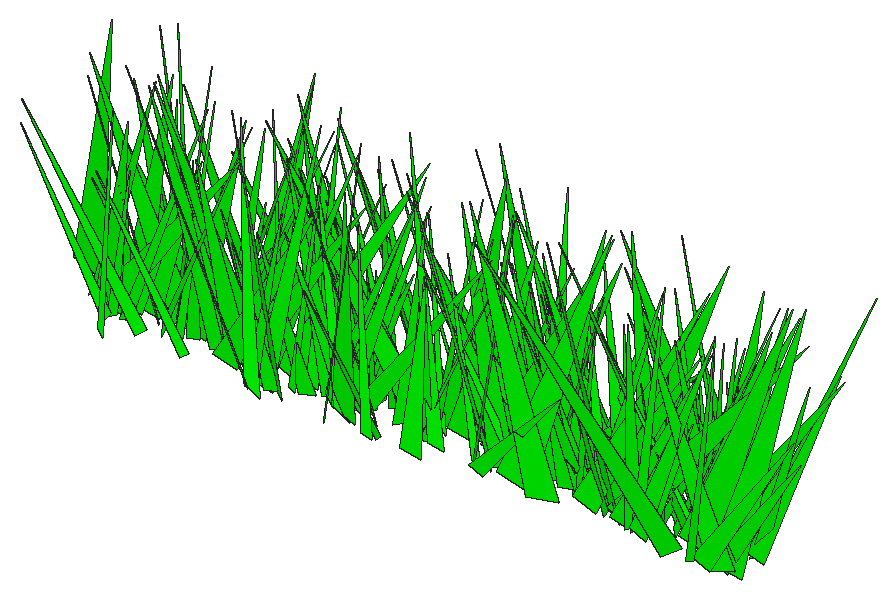
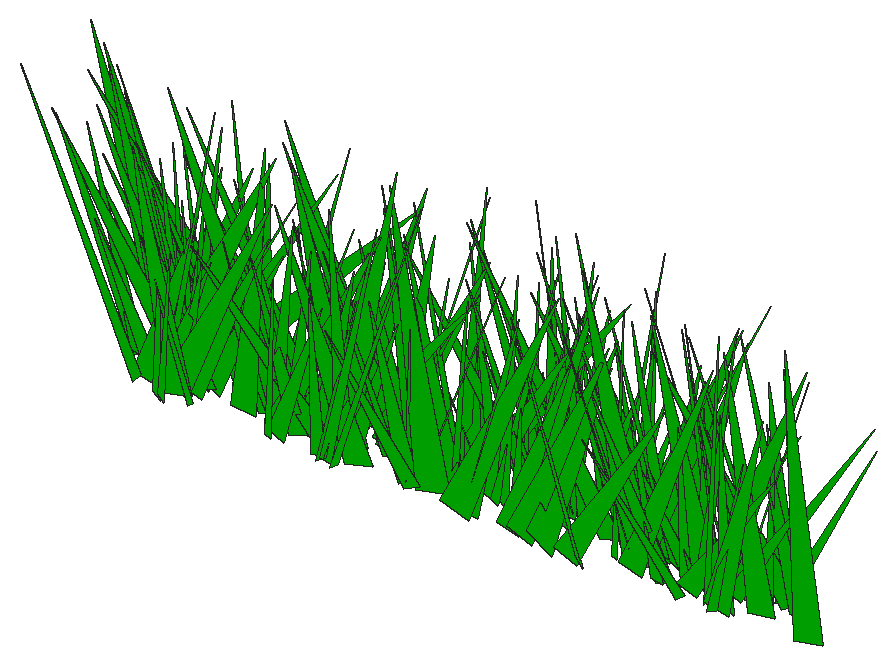
# SketchUp Ruby script. Lengths in inches.
U = 1.inch
M = Sketchup.active_model
def pt(a) = Geom::Point3d.new(a.map { |v| v * U })
def face(e, loops, mat)
  f = e.add_face(loops[0].map { |a| pt(a) })
  loops[1..].each { |l| e.add_face(l.map { |a| pt(a) }).erase! }
  f.material = f.back_material = mat if mat
  f
end
# faces: each face lists its corners as indices into pts; further lists are holes
def faces(e, pts, list, mat = nil) = list.each { |f| face(e, (f[0].is_a?(Array) ? f : [f]).map { |l| l.map { |i| pts[i] } }, mat) }
# xy, xz, yz: faces in a plane at the given z, y or x. An outline is a flat list of corners, or four numbers for a rectangle; further outlines are holes
def ring(l) = l.size == 4 ? [[l[0], l[1]], [l[2], l[1]], [l[2], l[3]], [l[0], l[3]]] : l.each_slice(2).to_a
def flat(e, list, mat, &to3) = list.each { |f| face(e, (f[0].is_a?(Array) ? f : [f]).map { |l| ring(l).map { |u, v| to3.(u, v) } }, mat) }
def xy(e, z, list, mat = nil) = flat(e, list, mat) { |x, y| [x, y, z] }
def xz(e, y, list, mat = nil) = flat(e, list, mat) { |x, z| [x, y, z] }
def yz(e, x, list, mat = nil) = flat(e, list, mat) { |y, z| [x, y, z] }
def lines(e, pts, list) = list.each { |a, b| e.add_line(pt(pts[a]), pt(pts[b])) }
# prism: a flat outline (further loops are holes) pulled along v
def prism(e, loops, v, mat = nil)
  f = face(e, loops, mat); d = Geom::Vector3d.new(v.map { |x| x * U })
  f.pushpull(f.normal.samedirection?(d) ? d.length : -d.length)
end
def box(e, o, s, mat = nil) = prism(e, [[o, [o[0] + s[0], o[1], o[2]], [o[0] + s[0], o[1] + s[1], o[2]], [o[0], o[1] + s[1], o[2]]]], [0, 0, s[2]], mat)
def at(x, y, z, deg = 0) = Geom::Transformation.translation(pt([x, y, z])) * Geom::Transformation.rotation(ORIGIN, Z_AXIS, deg.degrees)
def axes(o, x, y, z) = Geom::Transformation.new([*x, 0, *y, 0, *z, 0, *pt(o).to_a, 1])
def part(name) = M.definitions.add(name)
# library, detail: a bought-in or finely detailed component or shape, given as its bounding box
def library(name, o, s) = part(name).tap { |d| box(d.entities, o, s) }
def detail(e, o, s) = box(e.add_group.entities, o, s)
def put(e, d, t, mat = nil) = e.add_instance(d, t).tap { |i| i.material = mat if mat }
def group(e, t, mat = nil) = e.add_group.tap { |g| g.transformation = t; g.material = mat if mat }.entities
root = M.entities
M.materials.add("[0065_Lime]").color = [0, 255, 0]
c1 = part("fur_instance\#9")
p = [[0.8125,0,1.79],[0.67,-0.02,1.48],[0,-0.11,0],[0,0.11,0]]
faces(c1.entities,p,[[0,1,2,3]])
put(root,c1,axes([147.4375,26.02,1.48],[-5.64516,0.3336,1.45571],[-2.08323,-0.82888,1.01979],[2.12109,0.07376,4.87587]),"[0065_Lime]")
put(root,c1,axes([145.2,25.94,1.48],[8.40795,0.23314,2.16306],[-1.12337,1.22283,-1.52742],[-2.92617,0.20046,6.80163]),"[0065_Lime]")
put(root,c1,axes([165.61,26.26,1.48],[2.66875,-0.65598,0.87046],[4.49426,0.28351,-1.95751],[1.65526,0.28786,3.91148]),"[0065_Lime]")
put(root,c1,axes([142.26,26.54,1.48],[-8.02336,-0.38155,1.65588],[2.34325,-1.15401,-1.39815],[2.45487,-0.14551,6.74656]),"[0065_Lime]")
put(root,c1,axes([147.97,26.21,1.48],[-3.82032,-0.24279,0.04351],[1.61672,-0.49536,1.29689],[-0.61201,0.20701,3.15435]),"[0065_Lime]")
put(root,c1,axes([140.84,26.17,1.48],[-9.03308,-0.11216,0.2971],[0.85058,-1.24949,1.30518],[0.21674,0.22922,7.25986]),"[0065_Lime]")
put(root,c1,axes([164,26.24,1.48],[-6.04067,-0.94159,0.54512],[5.82851,-0.66764,4.0909],[-3.37327,0.53256,6.0923]),"[0065_Lime]")
put(root,c1,axes([132.93,25.9375,1.48],[6.59499,0.11964,2.32533],[0.40682,0.92959,-2.36602],[-2.95495,0.39499,4.86404]),"[0065_Lime]")
put(root,c1,axes([149.88,26.03,1.48],[-2.46962,0.72649,0.09041],[-5.01732,-0.34081,1.08686],[1.2525,0.06724,4.53207]),"[0065_Lime]")
put(root,c1,axes([166.41,26.53,1.48],[1.55477,-0.64987,0.45687],[4.2566,0.16434,-1.75131],[1.89367,0.16417,3.5615]),"[0065_Lime]")
put(root,c1,axes([145.53,26.86,1.48],[-4.02699,-0.94749,0.69367],[6.4082,-0.57572,-1.73659],[2.26451,-0.05572,6.14783]),"[0065_Lime]")
put(root,c1,axes([165.06,26.21,1.48],[5.85886,0.44745,1.24971],[-2.77667,0.84099,-1.47688],[-2.18863,0.13084,5.21912]),"[0065_Lime]")
put(root,c1,axes([166.75,26.49,1.48],[4.8644,-1.02334,2.31887],[7.81718,0.62202,-1.65156],[0.23532,0.49069,6.92962]),"[0065_Lime]")
put(root,c1,axes([153,26.61,1.48],[1.4391,-0.53575,0.3117],[3.28378,0.14278,-1.80769],[1.97492,0.15299,2.77859]),"[0065_Lime]")
put(root,c1,axes([166.7,26.33,1.48],[-0.36588,0.97693,0.95814],[-6.61726,0.00969,-2.00296],[-2.43605,-0.17305,5.2969]),"[0065_Lime]")
put(root,c1,axes([141.83,26.59,1.48],[-0.87819,0.53517,1.2943],[-4.04294,-0.06547,-0.90793],[-0.83171,-0.24685,3.04683]),"[0065_Lime]")
put(root,c1,axes([161.35,26.99,1.48],[5.61176,-0.59224,0.98641],[3.69096,0.78723,1.94481],[-2.36877,-0.17641,5.36723]),"[0065_Lime]")
put(root,c1,axes([140.88,26.33,1.48],[4.48129,0.51069,0.59791],[-3.46872,0.63464,-0.96252],[-1.31015,0.06651,4.59344]),"[0065_Lime]")
put(root,c1,axes([161.59,26.88,1.48],[7.74697,-0.349,1.60374],[2.08853,1.11185,1.4325],[-2.38618,-0.1599,6.4605]),"[0065_Lime]")
put(root,c1,axes([136.96,26.68,1.48],[-4.984,0.24551,0.07444],[-1.70865,-0.67466,-1.13],[-0.37633,-0.18835,4.14467]),"[0065_Lime]")
put(root,c1,axes([161.91,26.58,1.48],[5.56732,0.62425,1.04416],[-4.62002,0.7629,1.01505],[-0.19699,-0.25004,5.70396]),"[0065_Lime]")
put(root,c1,axes([141.14,26.09,1.48],[-7.77453,0.56542,0.94324],[-3.24423,-1.03052,3.00741],[2.64778,0.39754,6.45445]),"[0065_Lime]")
put(root,c1,axes([156.8,26.42,1.48],[-3.08785,1.12183,0.63152],[-7.94819,-0.41219,-1.17791],[-1.08012,-0.17399,6.8624]),"[0065_Lime]")
put(root,c1,axes([160.16,27.18,1.48],[-7.86104,-0.49414,0.8507],[3.15967,-1.08846,-1.8675],[1.86452,-0.23881,6.75137]),"[0065_Lime]")
put(root,c1,axes([162.06,26.87,1.48],[0.97601,0.53268,0.98411],[-3.85048,0.08226,1.03467],[1.00404,-0.20235,3.01129]),"[0065_Lime]")
put(root,c1,axes([141.33,26.65,1.48],[7.67947,-0.409,2.57949],[3.83398,1.06422,-1.89784],[-1.95674,0.48005,6.40494]),"[0065_Lime]")
put(root,c1,axes([134.26,27.0625,1.48],[-6.31802,0.34307,0.15568],[-2.36186,-0.83392,-1.83988],[-0.64737,-0.30573,5.19324]),"[0065_Lime]")
put(root,c1,axes([132.29,27.18,1.48],[-5.7439,0.16632,0.63301],[-1.40329,-0.73048,-1.99336],[0.19352,-0.36028,4.33389]),"[0065_Lime]")
put(root,c1,axes([149.61,27.23,1.48],[3.42726,-0.63133,0.5169],[4.34896,0.48895,0.93266],[-1.29478,-0.02881,4.50087]),"[0065_Lime]")
put(root,c1,axes([146.79,27.45,1.48],[-7.7596,-0.29508,0.73014],[1.64009,-1.0309,-2.4285],[1.58926,-0.37688,6.07112]),"[0065_Lime]")
put(root,c1,axes([153.12,27.42,1.48],[-8.76638,-0.23503,1.12036],[1.1973,-1.19774,-2.22109],[1.80588,-0.34682,6.91119]),"[0065_Lime]")
put(root,c1,axes([164.7,27.49,1.48],[-7.0411,-0.14326,0.04768],[0.87338,-0.87452,-2.71306],[0.52923,-0.46282,5.11168]),"[0065_Lime]")
put(root,c1,axes([160.48,26.92,1.48],[6.16842,-0.35486,0.6177],[2.63703,0.82834,-1.47766],[0.01656,0.27666,5.21644]),"[0065_Lime]")
put(root,c1,axes([154.93,26.82,1.48],[1.78992,1.23046,1.30776],[-8.68648,0.19085,1.84915],[1.95163,-0.27906,7.03096]),"[0065_Lime]")
put(root,c1,axes([164.53,27.29,1.48],[2.7894,-1.18504,1.60945],[8.4666,0.31122,-2.03016],[1.83137,0.36617,6.93425]),"[0065_Lime]")
put(root,c1,axes([160.5,27.17,1.48],[5.65586,-1.02642,0.41472],[6.57896,0.67259,-3.58382],[3.21463,0.4294,6.60486]),"[0065_Lime]")
put(root,c1,axes([138.63,27.33,1.48],[3.13442,-0.82289,0.38541],[5.65972,0.40265,-1.64714],[1.57692,0.19052,5.14568]),"[0065_Lime]")
put(root,c1,axes([152.6,26.92,1.48],[7.66984,0.18004,1.81115],[-0.72498,1.09679,-1.62211],[-2.46451,0.23767,6.11367]),"[0065_Lime]")
put(root,c1,axes([145.4375,27.32,1.48],[-3.7986,0.4408,1.09646],[-3.41146,-0.47842,-1.37489],[-0.13958,-0.30316,3.76399]),"[0065_Lime]")
put(root,c1,axes([143.2,27.29,1.48],[-1.07957,-0.60979,1.01436],[4.40538,-0.10276,1.03223],[-0.98978,0.20775,3.48793]),"[0065_Lime]")
put(root,c1,axes([132.35,27.46,1.48],[4.56281,-0.30782,0.7376],[1.97481,0.64636,0.95619],[-1.31199,-0.09764,4.00446]),"[0065_Lime]")
put(root,c1,axes([164.34,27.33,1.48],[2.99198,0.94609,2.07029],[-7.12124,0.33271,1.71453],[1.04751,-0.44042,5.74251]),"[0065_Lime]")
put(root,c1,axes([158.48,27.2,1.48],[5.63155,0.91693,0.33323],[-6.43994,0.76478,1.49277],[1.12939,-0.21126,6.85041]),"[0065_Lime]")
put(root,c1,axes([159.73,27.11,1.48],[-6.51852,-0.15935,1.07382],[1.55347,-0.85697,1.97799],[0.78457,0.37285,5.00523]),"[0065_Lime]")
put(root,c1,axes([139.23,27.64,1.48],[2.06806,-0.80807,1.15375],[5.54406,0.33839,1.36663],[-2.08452,0.09831,4.77938]),"[0065_Lime]")
put(root,c1,axes([152.63,27.12,1.48],[-5.92962,0.27492,0.83885],[-1.58432,-0.81735,1.56625],[1.54312,0.21723,4.83146]),"[0065_Lime]")
put(root,c1,axes([150.375,27.12,1.48],[-8.41795,0.48734,1.86206],[-3.09447,-1.22016,1.44482],[2.77362,0.11778,7.26333]),"[0065_Lime]")
put(root,c1,axes([162.33,27.7,1.48],[-4.37627,-0.25835,0.82463],[1.37909,-0.60204,-1.47796],[1.58312,-0.18972,3.56705]),"[0065_Lime]")
put(root,c1,axes([145.47,26.85,1.48],[-6.56106,0.53487,0.02483],[-3.40338,-0.82811,2.72507],[1.70487,0.40527,5.53555]),"[0065_Lime]")
put(root,c1,axes([149.31,27.18,1.48],[6.3211,0.24857,0.10937],[-1.7101,0.87235,-1.04106],[-0.47198,0.16823,5.23672]),"[0065_Lime]")
put(root,c1,axes([158.86,27.6875,1.48],[2.9523,-0.86442,0.1452],[5.81439,0.38266,-1.88462],[2.0169,0.16218,5.22051]),"[0065_Lime]")
put(root,c1,axes([142.41,27.23,1.48],[6.62121,0.01964,1.93094],[0.51715,0.95136,-1.49761],[-2.32107,0.26801,5.17462]),"[0065_Lime]")
put(root,c1,axes([134.81,27.86,1.48],[8.46994,0.06297,0.82168],[-0.78908,1.11274,2.52423],[-0.7737,-0.44551,6.42084]),"[0065_Lime]")
put(root,c1,axes([164.34,27.47,1.48],[-7.44728,-0.57469,0.22605],[4.01613,-1.00668,1.78436],[-0.82117,0.28849,6.67674]),"[0065_Lime]")
put(root,c1,axes([143.99,27.68,1.48],[7.23942,0.33066,0.96563],[-2.60144,0.97477,1.7191],[-0.42338,-0.33538,5.9485]),"[0065_Lime]")
put(root,c1,axes([164.99,27.69,1.48],[5.47269,0.35129,2.29874],[-3.2335,0.7972,1.01104],[-1.94449,-0.33696,4.78847]),"[0065_Lime]")
put(root,c1,axes([145.93,27.46,1.48],[6.17289,-0.51852,0.10712],[3.49429,0.80868,-2.05906],[1.19326,0.31425,5.4755]),"[0065_Lime]")
put(root,c1,axes([154.57,27.62,1.48],[-6.04014,0.24067,0.01901],[-1.67645,-0.82815,-1.11321],[-0.35141,-0.18589,4.98402]),"[0065_Lime]")
put(root,c1,axes([163.05,27.7,1.48],[8.69035,0.1972,0.7216],[-1.54084,1.20534,1.24009],[-0.61827,-0.23213,7.05222]),"[0065_Lime]")
put(root,c1,axes([147.87,27.8,1.48],[6.47371,-0.40288,1.26881],[2.65811,0.93329,0.9568],[-1.89417,-0.06723,5.67909]),"[0065_Lime]")
put(root,c1,axes([162.66,27.26,1.48],[-4.90919,0.12223,1.58395],[0.10525,-0.67199,1.95345],[2.13014,0.31489,3.55391]),"[0065_Lime]")
put(root,c1,axes([131.71,27.99,1.48],[-1.0198,-0.96221,0.16293],[6.69974,-0.14602,-1.15122],[1.42933,-0.00206,5.51241]),"[0065_Lime]")
put(root,c1,axes([164.97,28.13,1.48],[4.99778,-0.74484,0.71097],[4.41345,0.6649,2.81426],[-3.06306,-0.25727,5.21501]),"[0065_Lime]")
put(root,c1,axes([164.55,27.82,1.48],[-7.12618,0.16246,2.31186],[-1.77144,-1.04241,-1.15815],[2.50533,-0.27495,5.75698]),"[0065_Lime]")
put(root,c1,axes([139.33,28,1.48],[-5.9754,0.04689,1.35538],[-1.06204,-0.77125,-2.20374],[1.32664,-0.4062,4.34067]),"[0065_Lime]")
put(root,c1,axes([145.1,27.62,1.48],[7.55979,-0.39225,1.28092],[3.02913,1.05967,-0.95478],[-1.04721,0.23349,6.48516]),"[0065_Lime]")
put(root,c1,axes([140.06,27.86,1.48],[-1.44202,-1.11306,1.41639],[7.75763,-0.11682,2.14957],[-2.36545,0.29544,6.18621]),"[0065_Lime]")
put(root,c1,axes([162.17,27.56,1.48],[6.86854,-0.14514,0.21373],[1.06483,0.94488,-1.13979],[-0.04597,0.20023,5.53362]),"[0065_Lime]")
put(root,c1,axes([139.34,27.81,1.48],[4.47166,-0.80513,0.12539],[5.44319,0.58788,-1.9451],[1.796,0.2229,5.58287]),"[0065_Lime]")
put(root,c1,axes([140.18,28.17,1.48],[-4.30339,-0.76489,0.06594],[5.17343,-0.57911,-1.70764],[1.6949,-0.17445,5.37975]),"[0065_Lime]")
put(root,c1,axes([164.35,28.13,1.48],[-2.95262,-0.68746,0.01108],[4.71441,-0.4004,-1.23574],[1.30747,-0.10872,4.48079]),"[0065_Lime]")
put(root,c1,axes([144.28,27.8,1.48],[-4.00598,0.72132,1.88564],[-5.61919,-0.53925,-0.9863],[0.38657,-0.36358,5.20383]),"[0065_Lime]")
put(root,c1,axes([157.91,27.86,1.48],[-2.63089,-0.55555,0.54443],[3.96638,-0.34402,0.91837],[-0.58907,0.16481,3.75213]),"[0065_Lime]")
put(root,c1,axes([165.38,27.92,1.48],[-2.68175,-1.033,2.7912],[7.36867,-0.52261,-1.79684],[3.39415,0.3184,6.10627]),"[0065_Lime]")
put(root,c1,axes([167.17,28.22,1.48],[6.16671,-0.45835,0.07339],[3.14021,0.84094,1.40885],[-0.88717,-0.20941,5.4969]),"[0065_Lime]")
put(root,c1,axes([133.03,27.54,1.48],[7.01099,0.49772,0.24096],[-3.42004,0.9697,-1.27799],[-0.96804,0.1788,6.26019]),"[0065_Lime]")
put(root,c1,axes([138.01,28.11,1.48],[1.05469,-1.04002,1.77745],[7.26646,0.2382,1.81753],[-2.59884,0.24394,5.80323]),"[0065_Lime]")
put(root,c1,axes([137.75,28.3,1.48],[7.70208,-0.22449,0.44794],[1.34915,1.03433,2.02137],[-1.01755,-0.32784,6.07064]),"[0065_Lime]")
put(root,c1,axes([138.97,28.08,1.48],[2.90531,-0.95521,2.84578],[6.66064,0.57442,1.96168],[-3.75313,0.27998,5.68429]),"[0065_Lime]")
put(root,c1,axes([157.64,27.72,1.48],[5.16593,0.38808,1.14164],[-2.45136,0.74654,-1.16446],[-1.89426,0.09226,4.62037]),"[0065_Lime]")
put(root,c1,axes([153.71,27.51,1.48],[2.61886,1.06793,0.70593],[-7.11579,0.38741,-2.17282],[-2.80685,0.01425,6.16707]),"[0065_Lime]")
put(root,c1,axes([157.07,27.84,1.48],[1.60133,0.75412,1.68735],[-5.37489,0.30403,-1.17819],[-2.05308,-0.20776,4.40053]),"[0065_Lime]")
put(root,c1,axes([158.12,27.78,1.48],[-1.26453,0.72123,0.14316],[-4.91527,-0.16258,-1.2798],[-1.48834,-0.07584,4.10492]),"[0065_Lime]")
put(root,c1,axes([131.51,27.97,1.48],[4.58418,-0.78942,0.72038],[5.24543,0.52509,-2.80386],[2.19797,0.39333,5.18891]),"[0065_Lime]")
put(root,c1,axes([145.19,27.88,1.48],[-5.008,-0.30159,1.33724],[2.55239,-0.68774,1.127],[0.89131,0.27492,4.28621]),"[0065_Lime]")
put(root,c1,axes([140.32,28.21,1.48],[-0.18295,-0.65403,0.5521],[4.54764,-0.00022,0.98846],[-1.20135,0.09878,3.65768]),"[0065_Lime]")
put(root,c1,axes([153.79,27.89,1.48],[-2.72187,0.99916,0.97386],[-6.91501,-0.31073,-2.10465],[-2.0436,-0.27934,5.82452]),"[0065_Lime]")
put(root,c1,axes([165.16,27.68,1.48],[5.1634,0.64495,0.68081],[-4.225,0.7208,-1.67974],[-1.97895,0.1439,5.36253]),"[0065_Lime]")
put(root,c1,axes([143.97,28.44,1.48],[6.81898,-0.58292,2.40029],[3.32371,1.03478,2.17337],[-3.85613,-0.1389,6.11784]),"[0065_Lime]")
put(root,c1,axes([140.36,28.23,1.48],[7.20229,0.52703,1.38236],[-4.10026,0.96213,1.84312],[-0.3782,-0.39444,6.34283]),"[0065_Lime]")
put(root,c1,axes([134.04,28.48,1.48],[-7.2909,-0.28854,0.78179],[1.67541,-0.99212,-1.93187],[1.52749,-0.28904,5.85053]),"[0065_Lime]")
put(root,c1,axes([152.87,28.24,1.48],[3.28457,-1.12437,1.42926],[7.89478,0.3634,-2.42473],[2.18759,0.37673,6.6046]),"[0065_Lime]")
put(root,c1,axes([149.19,28.01,1.48],[-5.47868,0.97083,0.06403],[-6.41873,-0.70991,-2.70173],[-2.55731,-0.29803,6.64403]),"[0065_Lime]")
put(root,c1,axes([149.38,28.39,1.48],[7.84204,-0.1853,1.39082],[1.00968,1.11469,1.20983],[-1.90871,-0.17167,6.35423]),"[0065_Lime]")
put(root,c1,axes([153.83,28.14,1.48],[-3.68316,0.45863,0.42034],[-3.2641,-0.48798,-1.08264],[-0.51524,-0.18711,3.8538]),"[0065_Lime]")
put(root,c1,axes([135.69,27.92,1.48],[7.18761,-0.03402,2.07842],[0.90262,1.03297,-1.49871],[-2.40267,0.28629,5.65457]),"[0065_Lime]")
put(root,c1,axes([138.47,27.82,1.48],[5.31584,0.75568,0.6616],[-5.19266,0.75267,-1.2025],[-1.6182,0.06716,6.03207]),"[0065_Lime]")
put(root,c1,axes([162.94,28.61,1.48],[2.37772,-0.73063,0.28743],[4.30602,0.30617,2.51034],[-2.9357,-0.14268,3.9149]),"[0065_Lime]")
put(root,c1,axes([146.28,28.01,1.48],[-3.66656,-0.15592,1.56645],[1.81178,-0.51205,1.09797],[1.28738,0.27655,2.91616]),"[0065_Lime]")
put(root,c1,axes([130.61,28.65,1.48],[7.56406,-0.54323,0.20946],[3.67234,1.03051,1.81116],[-1.23506,-0.26284,6.66812]),"[0065_Lime]")
put(root,c1,axes([144.53,27.83,1.48],[4.48812,0.34143,0.76123],[-1.7608,0.59103,-2.0141],[-1.91814,0.25633,3.63004]),"[0065_Lime]")
put(root,c1,axes([142.9,27.98,1.48],[8.13305,-0.1707,2.75396],[1.99242,1.19306,-1.41519],[-2.99479,0.33017,6.5375]),"[0065_Lime]")
put(root,c1,axes([164.4375,28.33,1.48],[4.93111,-0.80973,0.02486],[5.39924,0.64724,-2.17571],[2.0137,0.24743,5.77278]),"[0065_Lime]")
put(root,c1,axes([167.125,28.1,1.48],[5.96096,-0.45577,1.20757],[3.56074,0.78451,-1.70779],[-0.21284,0.36008,5.24921]),"[0065_Lime]")
put(root,c1,axes([136.32,28.07,1.48],[3.67927,0.53598,1.12261],[-3.60315,0.5521,-1.01947],[-1.86312,-0.00927,4.18851]),"[0065_Lime]")
put(root,c1,axes([132.75,28.09,1.48],[4.08733,0.41532,1.4024],[-2.63903,0.62286,-1.09195],[-2.17801,0.0247,3.95488]),"[0065_Lime]")
put(root,c1,axes([135.91,28.47,1.48],[-0.83972,-1.01141,1.83728],[7.21471,-0.20097,-1.5254],[2.20388,0.27253,5.69364]),"[0065_Lime]")
put(root,c1,axes([149.45,28.73,1.48],[6.38288,-0.57279,0.01363],[3.95822,0.87195,1.45155],[-0.97422,-0.2101,5.98691]),"[0065_Lime]")
put(root,c1,axes([156.22,28.09,1.48],[0.92957,0.85814,1.03716],[-5.91327,0.17893,-1.45435],[-1.98852,-0.13094,4.80963]),"[0065_Lime]")
put(root,c1,axes([141.28,28.24,1.48],[6.28153,0.90093,0.49971],[-6.27148,0.82806,2.13418],[1.46739,-0.31759,6.98214]),"[0065_Lime]")
put(root,c1,axes([158.46,28.04,1.48],[6.04635,0.58342,0.29815],[-4.04338,0.84304,-1.025],[-1.01188,0.11743,5.87737]),"[0065_Lime]")
put(root,c1,axes([158.92,28,1.48],[-5.48107,0.48541,0.16941],[-3.10747,-0.71444,2.07564],[1.52323,0.28916,4.844]),"[0065_Lime]")
put(root,c1,axes([155.8,28.41,1.48],[-4.59274,0.72318,0.08427],[-4.72268,-0.58421,-2.30104],[-2.04798,-0.2746,5.11727]),"[0065_Lime]")
put(root,c1,axes([159.31,28.65,1.48],[3.73973,-1.16777,1.17355],[8.24658,0.45961,-2.06207],[1.7719,0.32558,7.12018]),"[0065_Lime]")
put(root,c1,axes([148.45,28.33,1.48],[-1.95659,0.84468,0.41906],[-5.65761,-0.23044,-1.91289],[-2.09562,-0.16651,4.77305]),"[0065_Lime]")
put(root,c1,axes([133.375,28.68,1.48],[1.4382,-0.75882,0.92124],[5.40431,0.16057,-1.15048],[1.11255,0.20097,4.39767]),"[0065_Lime]")
put(root,c1,axes([150.41,28.67,1.48],[0.72333,-0.72143,1.09467],[5.20522,0.05914,-0.96978],[1.03697,0.20638,4.10434]),"[0065_Lime]")
put(root,c1,axes([147.18,28.83,1.48],[-7.89157,0.02751,1.56222],[-0.69093,-1.10074,-1.65978],[1.80265,-0.30147,6.20286]),"[0065_Lime]")
put(root,c1,axes([132.66,28.47,1.48],[0.82493,0.6728,0.9197],[-4.7453,0.0663,1.19087],[1.29829,-0.18516,3.76832]),"[0065_Lime]")
put(root,c1,axes([135.12,28.97,1.48],[3.67498,-0.97908,1.99106],[6.0604,0.61937,2.80465],[-4.22037,0.03685,5.76119]),"[0065_Lime]")
put(root,c1,axes([145.55,28.92,1.48],[-5.59883,-0.44241,0.65062],[2.92632,-0.78413,-1.20537],[1.41034,-0.1293,5.0839]),"[0065_Lime]")
put(root,c1,axes([155.49,28.9,1.48],[6.41673,-0.12832,0.77194],[0.62124,0.87974,1.48348],[-1.16128,-0.23839,5.05902]),"[0065_Lime]")
put(root,c1,axes([134.0625,28.86,1.48],[-0.06481,-0.60284,0.18659],[3.82472,0.00659,1.59218],[-1.9569,0.03284,3.10571]),"[0065_Lime]")
put(root,c1,axes([145,28.4,1.48],[6.75265,-0.18204,1.28662],[1.78025,0.90069,-1.91176],[-1.00546,0.37217,5.25598]),"[0065_Lime]")
put(root,c1,axes([136.46,29.13,1.48],[4.29022,-0.41742,0.01984],[2.6473,0.53994,1.90024],[-1.34782,-0.26814,3.79549]),"[0065_Lime]")
put(root,c1,axes([144.71,28.91,1.48],[1.65626,-0.63549,0.32196],[4.40555,0.21071,-1.05905],[1.09564,0.11341,3.7717]),"[0065_Lime]")
put(root,c1,axes([155.0625,28.75,1.48],[-0.10978,-1.03012,2.85408],[7.90193,-0.12885,-1.35732],[1.90087,0.47616,5.80721]),"[0065_Lime]")
put(root,c1,axes([151.17,29.16,1.48],[6.8725,-0.58821,0.72056],[3.90105,0.95813,1.59133],[-1.7577,-0.17339,6.34915]),"[0065_Lime]")
put(root,c1,axes([165.55,28.62,1.48],[-2.80972,1.16363,1.0046],[-8.02651,-0.32226,-2.34502],[-2.38253,-0.28661,6.71542]),"[0065_Lime]")
put(root,c1,axes([136.09,29.06,1.48],[0.44866,-0.57721,0.25426],[3.58711,0.03301,-1.67692],[2.02584,0.06939,2.91297]),"[0065_Lime]")
put(root,c1,axes([146.89,28.71,1.48],[5.68555,0.55524,2.35403],[-3.66748,0.8956,-1.2178],[-3.24628,-0.03935,5.49866]),"[0065_Lime]")
put(root,c1,axes([149.65,28.48,1.48],[-6.42041,0.26537,1.21148],[-1.1009,-0.85467,2.41305],[2.13842,0.35676,4.87964]),"[0065_Lime]")
put(root,c1,axes([163.14,28.83,1.48],[4.4203,0.9306,1.07425],[-6.64903,0.56098,1.81797],[1.18065,-0.32488,6.21627]),"[0065_Lime]")
put(root,c1,axes([151.78,28.7,1.48],[-2.51968,0.86835,1.56021],[-5.94177,-0.42503,1.5778],[2.56181,-0.13173,5.19405]),"[0065_Lime]")
put(root,c1,axes([165.99,28.77,1.48],[0.26586,0.62278,0.46435],[-4.21318,0.00815,1.2296],[1.48922,-0.08811,3.39578]),"[0065_Lime]")
put(root,c1,axes([155.6,29.12,1.48],[2.93691,-0.65651,1.98987],[4.33079,0.52476,1.57224],[-3.00946,0.11448,4.20444]),"[0065_Lime]")
put(root,c1,axes([163.36,28.67,1.48],[4.78594,0.59584,0.10472],[-4.1331,0.66105,-1.05687],[-0.95616,0.12494,5.09259]),"[0065_Lime]")
put(root,c1,axes([159.84,28.7,1.48],[4.83067,0.39911,0.29655],[-2.60071,0.65351,-1.44188],[-1.19849,0.19054,4.32413]),"[0065_Lime]")
put(root,c1,axes([164.16,28.77,1.48],[-4.34909,0.36907,0.32619],[-2.31876,-0.58,1.53486],[1.29723,0.20063,3.8371]),"[0065_Lime]")
put(root,c1,axes([160.6,29.27,1.48],[5.1136,-0.81184,2.3777],[5.81892,0.80576,0.93881],[-2.83977,0.18917,6.20524]),"[0065_Lime]")
put(root,c1,axes([151.11,28.79,1.48],[-7.99907,0.10559,0.54726],[-0.52878,-1.08255,1.8851],[0.85888,0.31689,6.25741]),"[0065_Lime]")
put(root,c1,axes([134.68,28.91,1.48],[7.62455,0.27396,1.84724],[-1.60477,1.11135,-1.14042],[-2.52648,0.12086,6.29906]),"[0065_Lime]")
put(root,c1,axes([163.55,28.92,1.48],[5.32122,-0.10938,2.15415],[1.63805,0.7756,-1.35755],[-2.22174,0.30986,4.15844]),"[0065_Lime]")
put(root,c1,axes([155.43,29.08,1.48],[2.70384,1.12503,3.16096],[-8.36712,0.51579,-1.41603],[-3.03208,-0.42011,6.72634]),"[0065_Lime]")
put(root,c1,axes([139.01,28.66,1.48],[8.68347,0.47932,1.19281],[-2.76706,1.18489,-2.62675],[-2.47572,0.35686,7.11956]),"[0065_Lime]")
put(root,c1,axes([146.1,28.71,1.48],[3.6315,0.48134,0.07767],[-2.60728,0.40079,-2.57194],[-2.22377,0.31614,3.14235]),"[0065_Lime]")
put(root,c1,axes([132.07,29.43,1.48],[-2.41843,-0.9783,1.7897],[6.88579,-0.41392,-1.42525],[2.42863,0.19937,5.82314]),"[0065_Lime]")
put(root,c1,axes([140.14,29.4,1.48],[-7.01238,-0.02286,2.50167],[-0.3919,-1.05935,-1.05121],[3.05478,-0.18838,5.60782]),"[0065_Lime]")
put(root,c1,axes([137.79,28.91,1.48],[8.08882,-0.00623,0.72577],[0.31393,1.0891,-2.00171],[-0.83637,0.34854,6.26777]),"[0065_Lime]")
put(root,c1,axes([164.61,29.55,1.48],[-8.5971,-0.03905,2.2145],[-0.47662,-1.22057,-1.94555],[2.6948,-0.34047,6.7207]),"[0065_Lime]")
put(root,c1,axes([135.88,28.87,1.48],[-8.21796,-0.26749,2.70292],[3.10676,-1.11201,2.56216],[2.23911,0.56119,6.36527]),"[0065_Lime]")
put(root,c1,axes([149.81,29.77,1.48],[-1.95251,-1.2725,0.6327],[8.69783,-0.29404,-2.05683],[2.63825,0.02763,7.24923]),"[0065_Lime]")
put(root,c1,axes([163.38,29.38,1.48],[-1.01332,-0.79083,1.242],[5.5381,-0.06231,1.66004],[-1.82616,0.24985,4.34516]),"[0065_Lime]")
put(root,c1,axes([164.23,29.03,1.48],[1.34674,0.60932,0.30073],[-4.08427,0.19574,-1.18773],[-1.50292,0.01408,3.49719]),"[0065_Lime]")
put(root,c1,axes([164.72,29.61,1.48],[0.11855,-0.64873,0.02499],[4.4379,0.0172,1.03504],[-1.27283,-0.00044,3.61114]),"[0065_Lime]")
put(root,c1,axes([155.625,29.15,1.48],[-4.4578,0.37731,0.96465],[-2.33755,-0.63958,1.23553],[1.77547,0.10528,4.0487]),"[0065_Lime]")
put(root,c1,axes([165.69,29.7,1.48],[0.11555,-0.81503,0.44235],[5.64081,0.03475,1.17068],[-1.45574,0.06997,4.57137]),"[0065_Lime]")
put(root,c1,axes([151.59,29.25,1.48],[-4.49314,0.21463,1.15521],[-1.07962,-0.64488,1.23652],[1.78449,0.15026,3.65678]),"[0065_Lime]")
put(root,c1,axes([145.08,29.5,1.48],[-5.99199,0.77103,1.74419],[-5.87724,-0.81193,-1.33198],[0.40518,-0.37482,6.47319]),"[0065_Lime]")
put(root,c1,axes([158.74,29.39,1.48],[-6.00695,0.68613,0.36518],[-4.86822,-0.82256,-1.19573],[-0.58676,-0.19962,6.1822]),"[0065_Lime]")
put(root,c1,axes([155.87,29.46,1.48],[3.05345,-0.69752,0.75523],[4.24478,0.2719,-2.94001],[2.73582,0.35663,3.71868]),"[0065_Lime]")
put(root,c1,axes([164.06,29.65,1.48],[-2.32702,-0.94102,1.35037],[6.65067,-0.24041,1.96901],[-1.83626,0.32178,5.4202]),"[0065_Lime]")
put(root,c1,axes([154.48,29.68,1.48],[-1.12846,-0.63928,0.92441],[4.60208,-0.11946,0.94877],[-0.89991,0.19072,3.69278]),"[0065_Lime]")
put(root,c1,axes([128.98,30.05,1.48],[-3.56099,-1.14092,1.05557],[7.75454,-0.53207,-1.96216],[2.73422,0.0231,6.93964]),"[0065_Lime]")
put(root,c1,axes([139.39,29.0625,1.48],[7.48176,0.37324,0.49316],[-2.11217,0.95187,-2.93855],[-1.72094,0.4544,5.7506]),"[0065_Lime]")
put(root,c1,axes([157.41,29.47,1.48],[-1.59268,0.66337,1.32876],[-4.56028,-0.29143,1.25877],[2.03948,-0.13359,3.85226]),"[0065_Lime]")
put(root,c1,axes([137.44,29.9,1.48],[4.17247,-0.36695,0.23363],[2.4733,0.57421,0.99483],[-0.88579,-0.12519,3.87828]),"[0065_Lime]")
put(root,c1,axes([156.41,29.27,1.48],[2.3873,0.86535,0.6082],[-5.69368,0.35034,-1.91616],[-2.46295,0.02889,5.01916]),"[0065_Lime]")
put(root,c1,axes([138.79,29.27,1.48],[-2.68012,1.21818,1.40452],[-8.41533,-0.42922,1.84982],[2.70539,-0.12833,7.1454]),"[0065_Lime]")
put(root,c1,axes([158.88,29.32,1.48],[-5.50918,0.59965,0.70746],[-4.04119,-0.77733,1.2564],[1.62371,0.09994,5.52741]),"[0065_Lime]")
put(root,c1,axes([138.96,29.8,1.48],[-4.27637,-0.8349,0.89888],[6.02491,-0.57405,1.09799],[-0.47353,0.23593,5.85249]),"[0065_Lime]")
put(root,c1,axes([143.42,30.45,1.48],[5.12199,-0.96571,0.20473],[5.53892,0.60543,4.00861],[-4.07619,-0.39079,5.70433]),"[0065_Lime]")
put(root,c1,axes([158.12,30.12,1.48],[2.65241,-0.62096,0.03122],[3.82188,0.32547,2.08868],[-2.21885,-0.18168,3.63499]),"[0065_Lime]")
put(root,c1,axes([153.75,29.91,1.48],[2.6986,-0.95574,0.73811],[6.69165,0.33623,-1.59881],[1.51865,0.2168,5.73327]),"[0065_Lime]")
put(root,c1,axes([137.05,29.77,1.48],[2.38256,0.65248,1.37947],[-4.7713,0.23433,1.73845],[1.29308,-0.33759,3.87291]),"[0065_Lime]")
put(root,c1,axes([151.37,29.54,1.48],[-2.31877,0.68518,0.97812],[-4.59243,-0.36461,1.3553],[2.03279,-0.04214,4.17758]),"[0065_Lime]")
put(root,c1,axes([151.3,29.97,1.48],[6.10251,0.30846,0.78388],[-2.39117,0.80983,1.63813],[-0.17282,-0.31278,5.01446]),"[0065_Lime]")
put(root,c1,axes([148.13,29.71,1.48],[-6.69206,-0.1886,0.78008],[1.54732,-0.91284,1.38731],[0.57179,0.26295,5.37568]),"[0065_Lime]")
put(root,c1,axes([135.94,29.7,1.48],[-1.93175,0.70947,0.09266],[-4.65117,-0.24326,-1.74575],[-1.96759,-0.12151,4.03581]),"[0065_Lime]")
put(root,c1,axes([155.35,30.53,1.48],[-4.87021,-0.48207,0.01394],[3.05102,-0.61051,-2.19821],[1.56879,-0.30922,4.31839]),"[0065_Lime]")
put(root,c1,axes([144.54,30.4375,1.48],[2.61505,-0.93343,1.39798],[5.82234,0.43862,2.60755],[-3.63061,0.03107,5.18861]),"[0065_Lime]")
put(root,c1,axes([134.7,29.875,1.48],[-8.04938,0.12743,2.41688],[-0.35442,-1.18969,1.32094],[3.08631,0.19574,6.45513]),"[0065_Lime]")
put(root,c1,axes([133.95,30.45,1.48],[-4.14776,-0.44351,0.18418],[2.90662,-0.55473,-1.45144],[1.25087,-0.18162,3.98338]),"[0065_Lime]")
put(root,c1,axes([155.67,30.33,1.48],[-2.36154,-0.56027,0.84207],[3.8289,-0.36039,-0.93028],[1.51952,0.03738,3.65282]),"[0065_Lime]")
put(root,c1,axes([165.91,29.95,1.48],[8.99386,-0.13031,0.73952],[1.09769,1.24048,-1.50839],[-0.69398,0.27333,7.19816]),"[0065_Lime]")
put(root,c1,axes([145.28,30.3,1.48],[1.02206,-0.78747,1.54839],[5.46623,0.22967,1.52668],[-2.26925,0.19856,4.37489]),"[0065_Lime]")
put(root,c1,axes([133.62,29.9375,1.48],[4.13381,0.6352,1.21476],[-4.36555,0.61664,-0.97541],[-1.89917,-0.03482,4.88624]),"[0065_Lime]")
put(root,c1,axes([163.62,29.96,1.48],[-2.37931,0.95082,1.75937],[-6.72545,-0.40471,1.31128],[2.28758,-0.2009,5.68509]),"[0065_Lime]")
put(root,c1,axes([154.54,30.67,1.48],[-8.79929,-0.46959,0.67348],[2.94782,-1.19255,-2.38051],[1.77874,-0.34667,7.27678]),"[0065_Lime]")
put(root,c1,axes([162.68,30.3,1.48],[4.5103,0.19611,0.72036],[-1.59974,0.60891,1.07231],[-0.41589,-0.21537,3.68762]),"[0065_Lime]")
put(root,c1,axes([133.94,30.18,1.48],[-0.34325,-0.8203,2.20226],[6.3071,0.03269,1.05846],[-1.27655,0.38209,4.63741]),"[0065_Lime]")
put(root,c1,axes([154.81,29.59,1.48],[-7.41916,0.71246,1.11088],[-4.09726,-0.99323,3.24012],[3.28405,0.37037,6.5521]),"[0065_Lime]")
put(root,c1,axes([150.74,30.03,1.48],[0.81677,0.65714,0.21215],[-4.17421,0.08525,1.78462],[2.12475,-0.08514,3.42446]),"[0065_Lime]")
put(root,c1,axes([147.27,30.33,1.48],[-5.92442,0.3284,1.60019],[-2.75863,-0.83424,-1.02057],[1.31226,-0.2711,5.07889]),"[0065_Lime]")
put(root,c1,axes([158.35,30.4,1.48],[4.34184,-0.20815,1.37784],[1.0784,0.64648,1.02425],[-1.97501,-0.10461,3.58828]),"[0065_Lime]")
put(root,c1,axes([141.05,30.69,1.48],[7.38866,-0.16127,0.31781],[0.86446,0.93853,2.66137],[-0.85004,-0.44735,5.46892]),"[0065_Lime]")
put(root,c1,axes([148.1,30.44,1.48],[-2.49983,-1.08144,1.06515],[7.57319,-0.28903,1.92658],[-1.89514,0.27149,6.29381]),"[0065_Lime]")
put(root,c1,axes([164.3,30.6,1.48],[4.31335,-0.3029,0.72262],[1.57538,0.57218,1.81491],[-1.71869,-0.2357,3.4771]),"[0065_Lime]")
put(root,c1,axes([135.79,30.34,1.48],[3.52757,0.41005,0.06633],[-2.52739,0.41998,1.93262],[1.46097,-0.26353,3.18315]),"[0065_Lime]")
put(root,c1,axes([164.03,30.64,1.48],[4.43768,-0.23851,1.0712],[0.85755,0.58605,2.02192],[-1.96975,-0.2822,3.29359]),"[0065_Lime]")
put(root,c1,axes([141.87,30.61,1.48],[-0.84716,-0.87659,0.06294],[5.76254,-0.10574,1.97023],[-2.39072,0.05575,4.7267]),"[0065_Lime]")
put(root,c1,axes([155.12,30.5,1.48],[-7.30784,0.19589,1.78123],[-1.79868,-1.04493,-1.03192],[1.87173,-0.23935,5.96285]),"[0065_Lime]")
